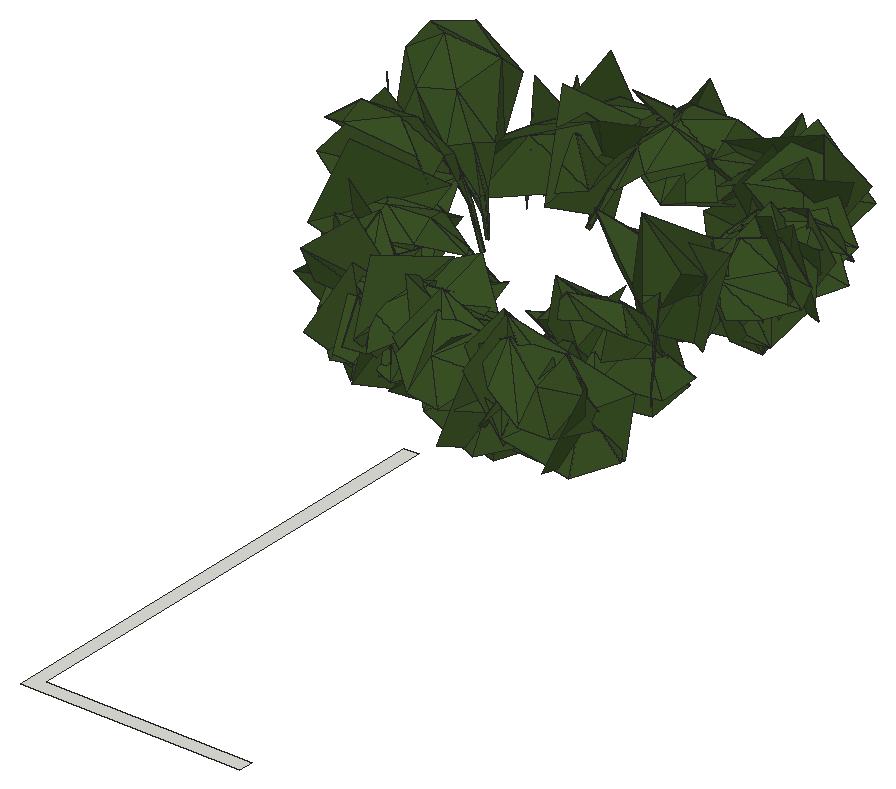
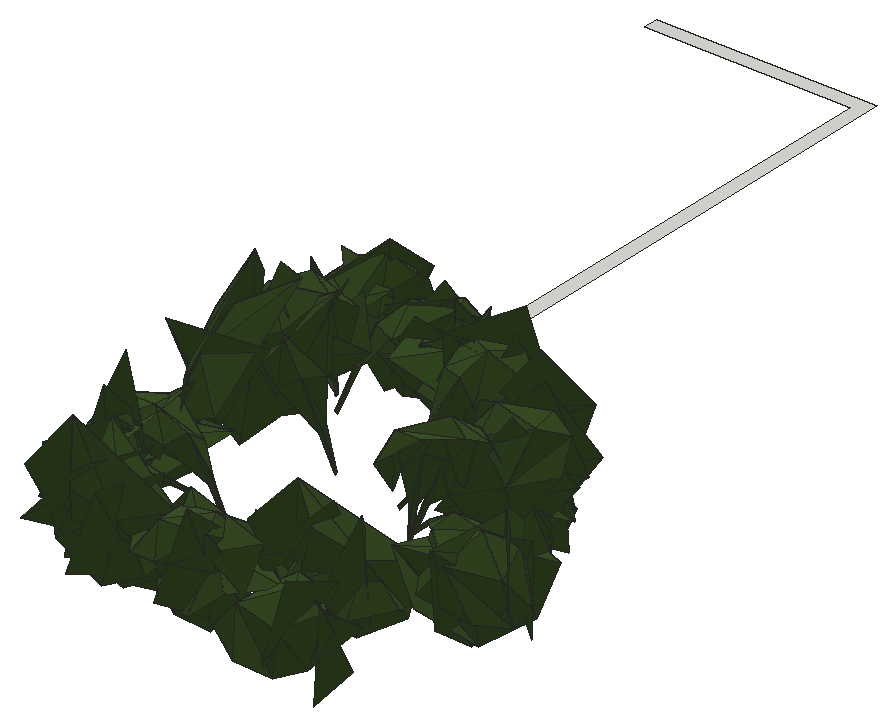
# SketchUp Ruby script. Lengths in inches.
U = 1.inch
M = Sketchup.active_model
def pt(a) = Geom::Point3d.new(a.map { |v| v * U })
def face(e, loops, mat)
  f = e.add_face(loops[0].map { |a| pt(a) })
  loops[1..].each { |l| e.add_face(l.map { |a| pt(a) }).erase! }
  f.material = f.back_material = mat if mat
  f
end
# faces: each face lists its corners as indices into pts; further lists are holes
def faces(e, pts, list, mat = nil) = list.each { |f| face(e, (f[0].is_a?(Array) ? f : [f]).map { |l| l.map { |i| pts[i] } }, mat) }
# xy, xz, yz: faces in a plane at the given z, y or x. An outline is a flat list of corners, or four numbers for a rectangle; further outlines are holes
def ring(l) = l.size == 4 ? [[l[0], l[1]], [l[2], l[1]], [l[2], l[3]], [l[0], l[3]]] : l.each_slice(2).to_a
def flat(e, list, mat, &to3) = list.each { |f| face(e, (f[0].is_a?(Array) ? f : [f]).map { |l| ring(l).map { |u, v| to3.(u, v) } }, mat) }
def xy(e, z, list, mat = nil) = flat(e, list, mat) { |x, y| [x, y, z] }
def xz(e, y, list, mat = nil) = flat(e, list, mat) { |x, z| [x, y, z] }
def yz(e, x, list, mat = nil) = flat(e, list, mat) { |y, z| [x, y, z] }
def lines(e, pts, list) = list.each { |a, b| e.add_line(pt(pts[a]), pt(pts[b])) }
# prism: a flat outline (further loops are holes) pulled along v
def prism(e, loops, v, mat = nil)
  f = face(e, loops, mat); d = Geom::Vector3d.new(v.map { |x| x * U })
  f.pushpull(f.normal.samedirection?(d) ? d.length : -d.length)
end
def box(e, o, s, mat = nil) = prism(e, [[o, [o[0] + s[0], o[1], o[2]], [o[0] + s[0], o[1] + s[1], o[2]], [o[0], o[1] + s[1], o[2]]]], [0, 0, s[2]], mat)
def at(x, y, z, deg = 0) = Geom::Transformation.translation(pt([x, y, z])) * Geom::Transformation.rotation(ORIGIN, Z_AXIS, deg.degrees)
def axes(o, x, y, z) = Geom::Transformation.new([*x, 0, *y, 0, *z, 0, *pt(o).to_a, 1])
def part(name) = M.definitions.add(name)
# library, detail: a bought-in or finely detailed component or shape, given as its bounding box
def library(name, o, s) = part(name).tap { |d| box(d.entities, o, s) }
def detail(e, o, s) = box(e.add_group.entities, o, s)
def put(e, d, t, mat = nil) = e.add_instance(d, t).tap { |i| i.material = mat if mat }
def group(e, t, mat = nil) = e.add_group.tap { |g| g.transformation = t; g.material = mat if mat }.entities
root = M.entities
M.materials.add("AM113_062_Tilia").color = [58, 81, 37]
xy(root,592.47,[[418.81,121.6875,695.48,121.6875,695.48,139.5,436.99,139.5,436.99,725.65,418.81,725.65]])
p = [[282.89,941.76,646.41],[303.81,882.98,547.76],[290.33,804.82,585.71],[153.17,1330.2,653.64],[148.44,1345.75,547.83],[160.28,1269.04,548.11],
  [236.98,1253.71,611.74],[267.24,972.73,609.64],[190.44,932.16,549.18],[149.66,888.95,626.87],[437.5,975.72,592.23],[421.98,970.82,549.59],
  [418.41,972.64,550.71],[516.82,1234.53,568.42],[468.37,1262.52,550.49],[475.61,1278.875,611.62],[436.02,1285.49,572.14],[433.9,975.55,598.71],
  [420.09,968.76,550.67],[434.63,969.11,602.37],[97.88,1159.51,551.17],[90.73,1088.16,561.68],[75.48,1108.44,636.62],[72.82,1166.52,632.64],
  [112.14,1207.35,675.32],[88.37,1230.22,603.9],[144.6,936.63,592.1875],[159.69,940.36,551.625],[254.46,938.14,555.38],[247.3125,855.98,551.82],
  [294.49,840.17,578.6],[255.06,867.5,631.61],[189.3,896.67,569.4375],[151.03,951.39,664.74],[125.57,972.41,565.63],[202.16,965.81,551.82],
  [242.93,1020.92,631.88],[246.7,860.73,682.55],[199.93,840.85,596.88],[264.52,866.93,552.73],[280.44,951.68,595.82],[173.95,1012.42,552.66],
  [189.03,1000.125,575.07],[85.13,1048.38,631.15],[93.0625,1053.85,587.64],[487.69,797.4,588.42],[540.59,838.35,553.52],[556.8125,836.77,632.54],
  [580.87,871.29,571.75],[157.92,958.01,554.29],[190.51,920.07,577.23],[184.18,968.24,627.41],[131.4,1024.91,578.625],[390.89,816.46,572.65],
  [461.64,813.46,554.71],[461.45,805.375,635.81],[510.1,814.44,585.16],[447.6,1283.55,584.17],[433.02,1276.21,554.78],[357.9375,1279.1,567.47],
  [528.87,1245.36,578.69],[483.3,1278.96,555.32],[472.13,1269.87,617.87],[446.8,1295.35,573.52],[266.99,936.89,584.83],[238.125,1043.32,650.45],
  [171.92,1059.68,558.42],[98.42,1034.5625,601.68],[511.17,1079.53,670.73],[554.79,1067.88,611.41],[540.93,1138.33,559.68],[547.43,1131.02,646.89],
  [530.15,1186.51,651.45],[528.09,1208.375,574.74],[490.18,1298.02,640.19],[455.49,1256.63,560.91],[452.05,1211.8125,636.5625],[511.89,1282.43,561.2],
  [573.45,818.58,674.68],[546.41,782.58,583.77],[538.83,857.81,561.15],[486.95,895.9,646.8],[85.01,1049.58,609.69],[80.41,1170.84,562.47],
  [64.8125,1098.21,567.67],[88.16,1110.94,641.78],[100.375,1166.56,645.96],[168.6875,1196.6,657.625],[112.58,1231.87,620.53],[456.51,782.58,679.1875],
  [426.69,767.83,580.21],[471.39,829.98,563.7],[443.59,895.78,639.46],[49.4375,1124.64,671.57],[46.14,1129.43,563.96],[105.48,1080.41,576.89],
  [495.58,781.4375,606.36],[553.96,815.67,566.49],[547.55,845.71,637.89],[588.14,855.24,578.3],[421.62,903.62,657.16],[375.09,851.67,567.07],
  [358.93,777.16,614.375],[349.86,1283.47,591.6],[68.3,1057.09,610.75],[384.25,799.88,590.5],[455.65,788.01,568.27],[459.26,818.36,639.79],
  [504.59,797.7,591.68],[525,1229.14,679.45],[560.46,1228.34,631.29],[517.25,1262.85,628.61],[206.64,894.46,654.63],[204.71,955.68,685.07],
  [150.52,934.82,649],[275.52,1227.68,615.29],[258.48,1212.95,572.02],[261.7,1214.78,569.39],[282.45,1228.62,613.99],[251.24,1156.23,616.69],
  [266.37,1246.74,569.84],[258.88,1297.7,656.41],[240.98,865.94,660.34],[247.33,827.32,594.29],[322.86,853.86,569.99],[300,838.26,650.56],
  [349.9,861.09,675.7],[385.3,872.95,609.62],[272.6,1231.36,610.09],[259.47,1216.6,569.98],[542.24,974.58,701.78],[573.52,920.77,629.74],
  [534.33,969.37,570.26],[447.48,972.45,611.05],[244.0625,1238.84,602.44],[259.37,1216.44,570.29],[261.75,1214.36,573.67],[247.47,1240.67,608.67],
  [262,1217.6875,570.32],[249.8,1247.18,606.78],[376.81,1253.75,675.28],[411.625,1289.14,622.27],[346.23,1318.76,570.53],[352.95,1313.4,657.96],
  [296.58,1327.74,661.32],[279.48,1343.68,585.32],[573.94,894.52,634.83],[428.91,1277.34,626.63],[405.63,799.9,656],[373.82,841.58,706.91],
  [337.12,809.61,652.42],[177.23,1234.1875,704.22],[169.29,1228.82,572.72],[226.36,1160.21,603.95],[189.58,1290.98,626.66],[464.92,1200.15,653.18],
  [513.42,1203.9,573.11],[556.53,1253.61,593.07],[416.73,1253.13,599.32],[521.98,893.74,607.61],[548.88,955.29,573.58],[534.61,972.87,649.96],
  [553.25,1008.05,586.7],[259.53,880.18,629.71],[283.1,830.44,592.26],[319.85,887.72,573.85],[226.15,993.55,633.36],[482.62,1307.05,592.23],
  [412.09,1313.89,574.65],[413.39,1325.3,655.0625],[363.89,1317.32,605.5],[513.3,1243.52,623.91],[171.39,1249.05,574.98],[130.05,1219.48,598.18],
  [176.66,1228.35,651.97],[239.54,1267.54,594.16],[146.89,1028.57,665.22],[178.85,1388.36,605.03],[191.26,1364.84,575.52],[184.82,1275.26,614.82],
  [232.61,840.87,575.94],[178.6,890.16,593.7],[521.28,973.97,647.35],[501.3,1020.79,576.92],[418.27,917.37,663.63],[565.06,1001.57,602.75],
  [166.11,1122.48,648.78],[460.22,1078.77,631.93],[529.01,1059.71,617.64],[557.28,1130.35,576.97],[518.92,1123.9,648.7],[517.85,1180.89,651.28],
  [553.15,1203.91,590.34],[408.68,1155.24,577.08],[435.09,1145.55,618.41],[430.76,1150.96,620.2],[405.67,1157.05,580.12],[251.79,950.33,593.78],
  [431.89,1155.3,614.71],[409.1,1158.11,577.55],[550.33,912.24,594.42],[314.75,874.75,626.38],[165.64,1018.17,653.71],[207.67,1078.99,671.25],
  [136.4,1080.97,656.2],[500.89,1189.24,669.35],[550.5625,1213.11,647.2],[505.625,1245.2,641.89],[240.56,919.82,628.78],[234.68,851.22,600.54],
  [314.18,835.19,581.99],[288.83,865.4,653.24],[342.82,872.61,675.08],[381.54,846.24,620.16],[550.26,1173.94,694.47],[509.13,1211.51,583.64],
  [446.83,1151.9375,626.85],[578.76,1178.01,593.19],[409.32,1278.22,636.38],[197.45,951.875,648.12],[420.11,1349.5,696.75],[401.36,1298.43,584.85],
  [425.41,1234.21,664.88],[450.09,1358.15,596.67],[510.27,839.48,647.71],[183.79,1217.25,648.13],[129.68,1233.04,614.1],[151.48,1170.9375,585.18],
  [293.39,1173.18,642.36],[240.21,1345.82,632.89],[300.125,836.65,691.92],[419.8,1339.42,586.38],[370.51,1333.92,610.8],[414.77,1312.39,659.93],
  [490.45,1323.89,608.85],[514.23,1027.25,629.22],[170.76,1381.52,586.95],[150.53,1352.3,590],[183,1361.58,627.5],[241.26,1352.28,635.34],
  [213.93,1390.3,596.15],[477.64,814.15,725.99],[462.42,763.12,679.17],[520.85,798.74,665.45],[429.71,957.37,628.8],[487.48,883.63,588.7],
  [537.46,866.92,674.0625],[446.96,1225.71,682.92],[496.08,1270.72,589],[517.35,1345.88,630.91],[467.86,889.26,670.01],[452.82,814.46,589.25],
  [494.05,749.37,634.3],[162.61,1307.55,631.6875],[150.125,1266.125,601.5],[194.875,1264.87,589.78],[200.79,1266.34,626.85],[361.03,1326.95,589.86],
  [343.93,1285.46,655.53],[351.93,1213.5,629.45],[404.8,1262.59,624.6],[294.88,1314.42,659.27],[295.9375,1361.2,604.28],[258.24,1026.05,621.66],
  [280.93,1041.88,590.28],[283.86,1042.93,593.74],[530.34,1239.85,631.26],[375.18,896.16,677.46],[337.53,835.25,665.15],[406.5,828.57,664.46],
  [280.45,1044.63,591.375],[252.18,1032.4375,629.42],[257.95,1028.37,629.05],[316.4,1334.625,706.65],[266.55,1328.64,591.54],[282.92,1241.22,624.2],
  [331.3125,1368.91,610.16],[509.38,866.36,604.37],[34.9,1183.33,616.75],[62.52,1173.17,592.14],[112.96,1103.7,644.13],[458.09,977.66,647.23],
  [481.4,986.42,631.88],[469.59,1327.98,674.42],[499.02,1286.49,727.91],[537.31,1313.7,671],[224.18,1043.9375,681.5],[183.27,985.9,593.07],
  [117.22,950.53,643.74],[508.41,1278.55,652.16],[513.02,1291.38,593.6],[445.89,1274.59,596.25],[476.9,1281.47,626.12],[522.54,1278.23,634.47],
  [539.55,1282.88,601.1],[221.44,919.63,649.95],[164.17,958.66,649.67],[216.24,1098.13,640.75],[220.21,1103.15,593.95],[224.17,1102.09,593.68],
  [221.04,1099.36,645.53],[221.82,1105.58,594.1875],[219.9,1105.75,649.13],[228.17,1247.3,677.04],[277.73,1208.26,700.41],[294.58,1266.72,672.99],
  [440.25,855.57,700.62],[234.06,1076.96,594.375],[210.76,1085.44,639.11],[217.7,1085.01,640.72],[237.67,1078.67,596.16],[447.06,911.21,628.41],
  [445.31,937.67,595.42],[445.85,940.84,598.71],[219.49,1079.34,638.53],[235.73,1075.05,596.23],[266.36,1356.22,602.67],[454.72,1239.8,604.8],
  [442.68,938.68,596.41],[438.39,909.48,636.1],[444.82,912.39,635.7],[248.69,1281.1,626.29],[259.1,1297.61,598.1],[145.1875,1177.9,639.36],
  [123.57,967.15,608.12],[206.9375,944.59,599.25],[173.29,959.55,641.32],[219.07,988.61,600.98],[35.21,1172.23,599.19],[39.19,1137.12,604.93],
  [53.42,1166.98,643.44],[101.93,1199.31,657.56],[60.48,1207.93,610.64],[544.5,1282.49,618.03],[531.9,1262.01,599.47],[458.19,1254.67,620.11],
  [191.92,1099.51,646.08],[132.27,1029.28,600.45],[73.15,1020.02,677.59],[530.33,888.9,633.97],[566.51,948.53,600.57],[222.51,986.82,638.53],
  [493.57,974.36,601.12],[529.81,976.86,666.88],[531.5625,998.75,610.1],[525.83,1236.11,662.16],[553.62,1255.94,625.16],[144.35,984.98,676.01],
  [169.01,1267.5,602.28],[241.41,1277.57,620.17],[444.33,954.1,644.4],[225.8,1271.02,640.63],[556.45,784.75,624.78],[563.875,869.43,603.1875],
  [559.31,837.4,650.98],[519.08,874.87,612.375],[514.05,981.65,637.79],[511.51,1048.77,603.76],[532.91,1059.76,679.41],[513.92,1100.66,622.35],
  [252.05,1357.66,642.54],[453.22,1243.78,634.57],[94.61,1073.27,629.37],[73.54,1113.39,654.05],[176.34,1270.03,645.91],[178.5,1351.75,682.05],
  [362.56,1294.98,669.71],[478.33,909.38,636.21],[455.77,926.85,606.14],[454.64,929.84,609.46],[448.37,784.01,693.36],[504.65,822.02,675.55],
  [459.14,913.72,718.63],[492.22,861,697.04],[518.84,924.39,686.26],[453.28,926.04,607.8125],[473.92,903.07,645.72],[476.91,909.33,643.98],
  [317.17,984.48,607.9375],[303.64,953.39,641.27],[307.88,958.09,645.34],[317.89,987.37,611.82],[126.68,991.92,655.73],[100.75,993.44,617.88],
  [255.93,857.05,650.69],[243.0625,864.7,608.64],[272.69,809.95,618.68],[276.23,913.01,619.17],[466.9375,1299.82,684.87],[493.93,1230.97,702.32],
  [535.34,1288.71,685.5],[97.96,998.84,639.14],[121.18,1011.15,609.17],[208.64,976.41,624.35],[313.25,958,641.39],[319.88,984.35,609.3],
  [407.48,886.75,670.46],[224.91,888.27,687.73],[104.18,1063.61,673.07],[565.62,933.17,668.44],[293.23,1251.14,658.85],[278.92,1274.29,652.96],
  [121.15,1217.91,626.72],[134.75,1052.77,636.57],[361.4,1266.34,628.29],[533.4375,977.51,651.77],[538.8125,1044.65,611],[520.98,1058.21,687.38],
  [531.55,1096.08,625.15],[461.05,805.07,654.53],[491.52,825.02,611.875],[459.71,857.8,611.06],[462.54,861.16,648.52],[332.41,835.72,710.4375],
  [359.77,817.81,611.16],[383.9375,891.13,621.45],[429.69,764.93,622.97],[442.98,1201.4,631.45],[432.06,1178.54,612.12],[430.57,1177.08,615.4],
  [590.17,1124.27,646.1875],[567.71,1129.85,612.1875],[492.61,1182.26,643.97],[524.3125,881.47,648.67],[472.61,1110.26,612.39],[516.33,1070.9,620.59],
  [522.71,1090.91,658.1],[461.2,1125.6875,640.93],[373.64,1270.49,664.64],[312.3,1238.35,639.63],[332.37,1242.12,612.53],[388.52,1257.56,625.99],
  [444.4,1200.7,637.49],[433.51,1176.94,613.25],[450.01,1200.11,637.42],[424.03,794.21,689.13],[299.66,795.43,642.59],[308.39,821.47,614.44],
  [341.99,898.35,671.49],[274.86,897.34,614.375],[291.52,893.73,639.84],[173.87,868.95,670.29],[182.02,882.01,629.64],[463.59,1148.9,659.39],
  [475.08,1173.1875,651.24],[562.5625,1060.8,715.78],[561.51,1017.73,623.33],[496.54,1059.67,614.84],[445.91,1043.05,712.33],[182.09,1115.86,642.42],
  [211.38,1108.38,615.26],[214.18,1108.54,619.13],[182.79,1119.7,648.61],[212.51,1111.07,615.33],[180.41,1126.03,645.94],[481.68,1182,616.12],
  [529.2,1180.84,668.65],[505.65,1216.95,638.11],[212.41,1233.73,708.59],[107.06,1095.2,675.01],[51.17,1158.53,698.59],[151.84,1042.7,678.32],
  [104.7,1033.96,641.46],[449.41,1266.16,639.46],[508.64,1290.82,672.39],[314.48,797.36,630.68],[283.9375,923.26,653.15],[276.09,1287.32,619.2],
  [300.33,1322.57,678.15],[258.28,1324.21,645.29],[404.9375,868.83,674.29],[238.63,1220.73,667.86],[304.78,1241.36,669.4],[573.76,1095.19,629.51],
  [309.79,941.72,650.17],[225.93,1008.46,660.19],[129.74,1101.86,621.75],[129.48,1108.17,658.76],[499.9,1109.57,689.41],[395.36,758.92,632.39],
  [409.34,781.8,669.25],[484.6,1220.97,676.24],[214.125,960.85,650.4],[535.58,759.12,641.89],[536.89,787.82,676.27],[466.47,1102.82,655.54],
  [536.97,1212.1,647.98],[397.8125,1318.08,643.6],[483.9,1257.76,653.51],[201.24,1309.22,648.4],[154.88,1169.39,630.47],[445.36,875.8125,669],
  [520.22,948.48,713.57],[383.72,935.03,676.7],[221.14,1035.17,655.54],[591.1875,1136.27,629.7],[226.65,1293.55,631.03],[563.08,1134.05,664.8],
  [577.79,1169.04,634.69],[461.93,1227.4375,629.78],[155.28,1151.14,660.03],[301.67,821.46,666.96],[343.06,813.77,648.11],[451.84,1336.21,707.24],
  [460.2,1229.88,654.74],[492.65,965.29,682.59],[378.07,829.95,688.43],[362.15,783.64,653.89],[242.52,1305.53,680.27],[465.92,868.77,694.875],
  [491.07,932.1,678.6],[542.95,807.83,693.1],[446.88,925.8,635.22],[461.32,883.3,684.95],[475.65,911.35,707.09],[205.64,1054.53,635.42],
  [151.9,1073.85,655.38],[419.97,885.04,663.29],[504.96,883.28,673.94],[473.76,1212.74,653.65],[512.49,983.5,777.62],[535.9,939.73,724.6],
  [543.58,1007.61,709.85],[491.23,1203.04,637.93],[159.04,1085.39,638.32],[100.92,1090.33,651.11],[112.17,1088.9,695.01],[179.61,1093.125,663.31],
  [183.49,992.64,669.12],[194.77,1084.11,690.32],[202.37,1058.65,699.93],[139.68,974.17,704.35],[317.5,1285.6875,681.79],[231,884.53,718.53],
  [209.73,1095.84,701.23],[186.19,1082.05,695.86],[507.45,1146.84,676.24],[302.98,921.73,678.44],[329.44,913.92,677.46],[485.6,806.69,706.03],
  [497.89,758.75,672.73],[143.56,1128.83,673.83],[342.3125,899.58,705.09],[294.04,829.04,721.52],[395.68,880.79,642.9],[351.53,844.97,664.05],
  [99.4,1141.03,673.64],[372.09,1354.44,647.23],[156.8,968.29,743.71],[489.0625,1189.52,675.96],[337.04,1360.03,651.05],[479.16,874.18,675.125],
  [345.56,911.76,645.91],[341.02,859.74,690.43],[378.2,889.95,676.04],[129.74,1056.01,752.69],[550.68,1138.66,718.45],[358.01,1326.76,678.06],
  [437.37,831.57,680.34],[528.32,844.63,683.88],[217.3,1121.27,692.56],[303.92,876.63,688.79],[76.05,1046.47,699.27],[454.27,980.99,764.36],
  [512.99,942,743.93],[516.98,1009.74,725.83],[371.77,907.49,716.49],[460.62,854.45,660.69],[452.7,800.26,689.58],[162.4,1068.11,726.69],
  [532.61,927.9,706.44],[559.09,902.19,689.48],[146.84,1084.71,747.71],[136.77,1059.45,694.83],[165.48,1089.75,670.9],[169.14,1030.9,746.37],
  [208.97,1007.96,723.74],[201.36,1035.08,677.35],[193.6,1161.28,763.31],[207.24,1147.97,684.02],[196.48,1190.03,735.88],[522.05,880.37,704.92],
  [182.875,1103.82,747.99],[105.01,1121.07,761.87],[91.24,1010.14,726.37],[112.42,1041.23,740.53],[123.58,998.14,737.81],[143.54,1183.02,778.36],
  [143.42,1134.6,785.19],[109.71,1153.91,778.57]]
faces(root,p,[[0,1,2],[3,4,5],[3,5,6],[7,8,9],[10,11,12],[13,14,15],[14,16,15],[17,12,18],
  [18,19,17],[12,17,10],[20,21,22],[22,23,20],[20,23,24],[24,25,20],[26,27,28],[29,30,31],
  [32,29,31],[33,34,35],[33,35,36],[37,38,39],[37,39,40],[41,42,43],[43,44,41],[45,46,47],
  [46,48,47],[49,50,51],[52,49,51],[53,54,55],[54,56,55],[57,58,59],[60,61,62],[61,63,62],
  [28,64,26],[65,66,67],[68,69,70],[70,71,68],[72,71,70],[70,73,72],[74,75,76],[74,77,75],
  [78,79,80],[78,80,81],[21,82,22],[83,84,85],[85,86,83],[83,86,87],[87,88,83],[89,90,91],
  [89,91,92],[93,94,95],[96,97,98],[97,99,98],[100,101,102],[59,103,57],[84,104,85],[105,106,107],
  [106,108,107],[109,110,13],[13,111,109],[15,111,13],[31,112,32],[32,112,113],[113,114,32],[115,116,117],
  [117,118,115],[119,120,121],[122,123,124],[124,125,122],[126,125,124],[124,127,126],[128,129,116],[130,131,132],
  [130,132,133],[134,135,136],[137,136,138],[138,139,137],[140,141,142],[142,143,140],[144,143,142],[142,145,144],
  [47,48,146],[116,115,128],[15,16,147],[53,148,149],[55,148,53],[149,150,53],[151,152,153],[151,154,152],
  [155,156,157],[62,63,158],[159,160,161],[160,162,161],[136,137,134],[163,164,165],[163,165,166],[167,168,169],
  [168,170,169],[73,171,72],[172,173,174],[175,172,174],[42,176,43],[177,178,179],[180,164,163],[181,180,163],
  [182,183,184],[182,185,183],[93,95,186],[187,188,189],[189,190,187],[191,190,189],[189,192,191],[193,194,195],
  [195,196,193],[51,50,197],[198,199,196],[98,99,200],[31,30,201],[51,202,52],[52,202,203],[203,204,52],
  [205,206,60],[60,207,205],[62,207,60],[196,195,198],[208,209,210],[210,211,208],[212,211,210],[210,213,212],
  [214,215,216],[214,217,215],[103,218,57],[64,219,26],[220,221,222],[220,223,221],[55,56,224],[225,226,227],
  [225,227,228],[145,229,144],[230,0,2],[231,232,233],[234,231,233],[161,162,235],[236,237,238],[239,240,236],
  [236,238,239],[241,242,45],[45,243,241],[47,243,45],[244,245,246],[247,248,249],[250,251,252],[253,254,255],
  [255,256,253],[257,258,259],[259,260,257],[261,258,257],[257,262,261],[237,254,253],[238,237,253],[263,264,265],
  [192,266,191],[267,268,105],[105,269,267],[107,269,105],[270,271,272],[272,265,270],[273,274,275],[273,276,274],
  [107,108,277],[278,279,280],[10,17,281],[281,282,10],[167,283,284],[284,285,167],[169,283,167],[286,287,288],
  [289,155,157],[290,291,292],[293,290,292],[294,290,293],[163,295,181],[166,296,181],[181,295,166],[265,272,263],
  [297,298,299],[299,300,297],[300,299,301],[51,197,203],[301,302,300],[175,303,304],[304,305,175],[174,303,175],
  [98,200,306],[307,308,309],[309,310,307],[311,312,313],[314,315,310],[310,309,314],[239,316,240],[292,291,317],
  [318,319,320],[320,313,318],[239,321,322],[322,316,239],[174,173,323],[313,320,311],[281,17,19],[324,325,326],
  [326,325,327],[328,329,330],[328,330,331],[331,332,328],[62,158,205],[333,334,335],[336,337,338],[339,340,182],
  [340,185,182],[327,341,326],[342,282,343],[343,344,342],[294,293,345],[345,346,294],[347,65,67],[348,226,225],
  [349,348,225],[19,350,281],[351,256,134],[134,137,351],[352,353,354],[354,353,355],[356,357,358],[357,359,358],
  [262,360,261],[107,277,267],[317,361,292],[329,362,363],[330,329,363],[179,364,177],[364,365,177],[169,170,366],
  [367,368,369],[306,370,96],[96,371,306],[98,371,96],[351,137,139],[139,321,351],[372,373,159],[159,374,372],
  [161,374,159],[375,376,377],[377,369,375],[378,379,380],[380,381,378],[382,324,326],[383,324,382],[384,385,386],
  [387,385,384],[234,388,389],[389,390,234],[233,388,234],[391,392,393],[394,395,381],[369,377,367],[127,396,126],
  [397,7,9],[22,82,398],[399,344,343],[128,115,400],[400,401,128],[331,402,332],[85,104,403],[233,232,404],
  [405,406,407],[406,408,407],[409,410,411],[411,412,409],[413,414,415],[15,147,109],[109,111,15],[381,380,394],
  [416,410,409],[417,418,419],[420,421,422],[355,423,354],[424,425,426],[426,427,424],[428,429,430],[430,431,428],
  [432,419,433],[433,434,432],[400,115,118],[118,429,400],[435,100,102],[436,437,438],[439,440,441],[441,442,439],
  [198,195,443],[443,444,198],[445,446,447],[445,447,448],[449,450,451],[452,451,453],[453,454,452],[419,432,417],
  [455,444,456],[456,457,455],[458,119,121],[280,459,278],[459,460,278],[383,382,461],[461,462,383],[205,207,62],
  [335,463,333],[463,464,333],[194,427,443],[443,195,194],[384,386,465],[451,452,449],[384,466,387],[467,401,468],
  [468,469,467],[213,470,212],[349,471,228],[228,472,349],[225,471,349],[426,425,473],[413,415,474],[475,341,263],
  [263,272,475],[363,362,476],[476,477,363],[358,359,478],[479,416,480],[480,416,409],[72,171,481],[393,482,391],
  [483,352,484],[484,352,354],[407,408,485],[345,486,346],[428,431,487],[488,292,361],[488,293,292],[489,351,321],
  [321,239,489],[31,201,113],[490,402,331],[489,253,256],[489,256,351],[203,202,51],[489,238,253],[239,238,489],
  [233,404,389],[491,412,311],[311,320,491],[208,211,212],[492,244,246],[212,493,208],[475,272,271],[161,235,372],
  [271,494,475],[426,473,495],[261,496,259],[259,258,261],[166,295,163],[495,497,426],[495,498,497],[191,499,187],
  [191,266,499],[331,500,490],[465,501,384],[465,502,501],[503,247,249],[261,360,496],[417,432,504],[504,361,417],
  [113,112,31],[505,282,281],[505,343,282],[187,190,191],[506,507,479],[479,480,506],[241,243,47],[47,146,241],
  [24,23,22],[144,229,508],[184,509,339],[339,510,184],[182,510,339],[511,250,252],[345,293,488],[488,361,504],
  [497,498,456],[498,457,456],[512,513,514],[514,350,512],[461,494,515],[515,516,461],[491,320,319],[149,148,55],
  [55,224,149],[319,517,491],[518,423,367],[367,377,518],[85,403,87],[22,398,24],[504,432,434],[434,519,504],
  [520,521,356],[356,522,520],[358,522,356],[306,371,98],[345,519,523],[523,486,345],[524,525,526],[526,527,524],
  [528,326,341],[528,341,475],[529,530,314],[314,309,529],[482,531,391],[308,527,529],[529,309,308],[174,323,304],
  [532,400,429],[429,428,532],[267,269,107],[440,533,441],[534,535,297],[297,300,534],[427,426,536],[536,443,427],
  [379,466,537],[537,380,379],[528,382,326],[537,538,394],[394,380,537],[461,516,462],[87,86,85],[539,540,483],
  [483,484,539],[541,477,449],[449,452,541],[228,471,225],[542,543,436],[438,542,436],[544,545,506],[506,517,544],
  [546,330,363],[331,330,546],[428,487,547],[548,286,288],[518,377,376],[422,549,420],[350,514,505],[505,281,350],
  [550,469,468],[534,300,302],[376,551,518],[552,538,553],[553,554,552],[541,452,454],[454,500,541],[555,336,338],
  [549,556,420],[68,71,72],[547,557,428],[547,550,557],[184,510,182],[501,502,553],[502,554,553],[558,409,412],
  [558,412,491],[559,354,423],[559,423,518],[302,560,534],[372,374,161],[122,125,126],[384,501,561],[466,384,561],
  [559,484,354],[557,550,468],[526,525,562],[536,444,443],[536,456,444],[72,481,68],[563,564,405],[405,565,563],
  [407,565,405],[304,303,174],[532,401,400],[532,468,401],[561,537,466],[488,504,519],[519,345,488],[506,545,507],
  [546,363,477],[558,480,409],[169,366,284],[284,283,169],[407,485,563],[494,461,528],[528,475,494],[461,382,528],
  [500,331,546],[140,143,144],[426,497,536],[546,477,541],[389,388,233],[546,541,500],[126,566,122],[567,568,539],
  [539,551,567],[144,508,140],[517,506,558],[558,491,517],[527,526,569],[569,529,527],[428,557,532],[536,497,456],
  [505,570,343],[570,399,343],[561,501,553],[571,399,570],[506,480,558],[126,396,566],[572,573,574],[574,535,572],
  [539,568,540],[559,518,551],[212,470,493],[551,539,559],[539,484,559],[575,576,577],[577,530,575],[561,553,538],
  [561,538,537],[532,557,468],[358,478,520],[520,522,358],[514,570,505],[578,560,579],[579,580,578],[514,513,581],
  [563,565,407],[514,581,571],[571,570,514],[569,530,529],[582,534,560],[560,578,582],[583,573,572],[526,562,584],
  [584,585,526],[526,585,569],[582,572,535],[582,535,534],[569,575,530],[586,576,575],[584,586,585],[569,585,575],
  [578,580,587],[585,586,575],[588,583,572],[582,588,572],[578,588,582],[589,583,588],[589,588,578],[578,587,589]],"AM113_062_Tilia")
